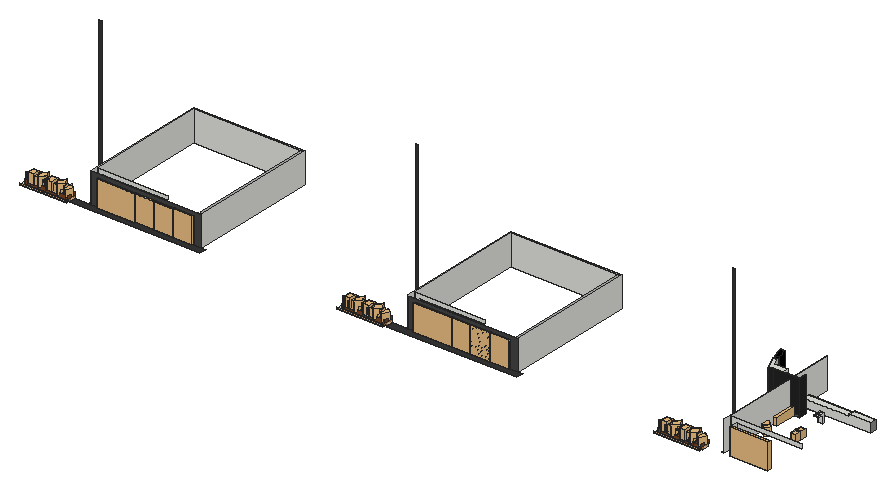
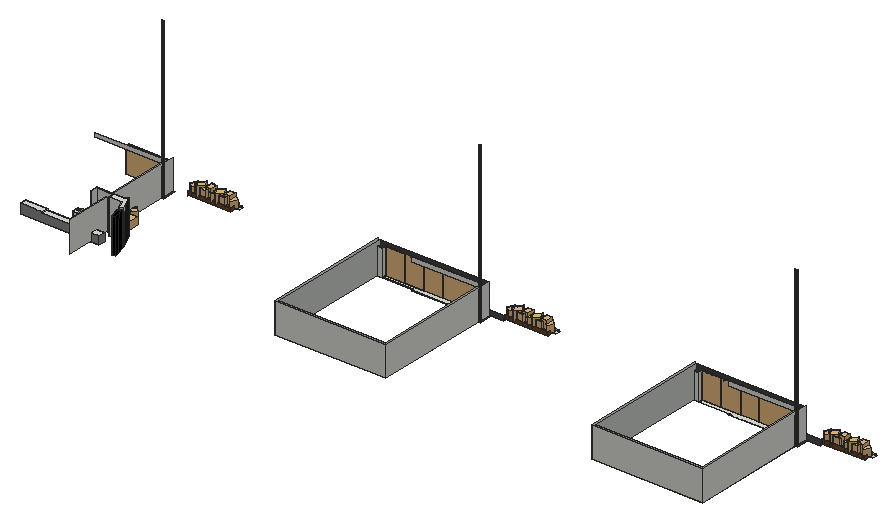
# SketchUp Ruby script. Lengths in inches.
U = 1.inch
M = Sketchup.active_model
def pt(a) = Geom::Point3d.new(a.map { |v| v * U })
def face(e, loops, mat)
  f = e.add_face(loops[0].map { |a| pt(a) })
  loops[1..].each { |l| e.add_face(l.map { |a| pt(a) }).erase! }
  f.material = f.back_material = mat if mat
  f
end
# faces: each face lists its corners as indices into pts; further lists are holes
def faces(e, pts, list, mat = nil) = list.each { |f| face(e, (f[0].is_a?(Array) ? f : [f]).map { |l| l.map { |i| pts[i] } }, mat) }
# xy, xz, yz: faces in a plane at the given z, y or x. An outline is a flat list of corners, or four numbers for a rectangle; further outlines are holes
def ring(l) = l.size == 4 ? [[l[0], l[1]], [l[2], l[1]], [l[2], l[3]], [l[0], l[3]]] : l.each_slice(2).to_a
def flat(e, list, mat, &to3) = list.each { |f| face(e, (f[0].is_a?(Array) ? f : [f]).map { |l| ring(l).map { |u, v| to3.(u, v) } }, mat) }
def xy(e, z, list, mat = nil) = flat(e, list, mat) { |x, y| [x, y, z] }
def xz(e, y, list, mat = nil) = flat(e, list, mat) { |x, z| [x, y, z] }
def yz(e, x, list, mat = nil) = flat(e, list, mat) { |y, z| [x, y, z] }
def lines(e, pts, list) = list.each { |a, b| e.add_line(pt(pts[a]), pt(pts[b])) }
# prism: a flat outline (further loops are holes) pulled along v
def prism(e, loops, v, mat = nil)
  f = face(e, loops, mat); d = Geom::Vector3d.new(v.map { |x| x * U })
  f.pushpull(f.normal.samedirection?(d) ? d.length : -d.length)
end
def box(e, o, s, mat = nil) = prism(e, [[o, [o[0] + s[0], o[1], o[2]], [o[0] + s[0], o[1] + s[1], o[2]], [o[0], o[1] + s[1], o[2]]]], [0, 0, s[2]], mat)
def at(x, y, z, deg = 0) = Geom::Transformation.translation(pt([x, y, z])) * Geom::Transformation.rotation(ORIGIN, Z_AXIS, deg.degrees)
def axes(o, x, y, z) = Geom::Transformation.new([*x, 0, *y, 0, *z, 0, *pt(o).to_a, 1])
def part(name) = M.definitions.add(name)
# library, detail: a bought-in or finely detailed component or shape, given as its bounding box
def library(name, o, s) = part(name).tap { |d| box(d.entities, o, s) }
def detail(e, o, s) = box(e.add_group.entities, o, s)
def put(e, d, t, mat = nil) = e.add_instance(d, t).tap { |i| i.material = mat if mat }
def group(e, t, mat = nil) = e.add_group.tap { |g| g.transformation = t; g.material = mat if mat }.entities
root = M.entities
M.materials.add("Material__1").color = [95, 70, 46]
M.materials.add("Sophie_Shoes2").color = [35, 35, 35]
M.materials.add("Sophie_Skirt").color = [0, 0, 0]
M.materials.add("Stain").color = [141, 140, 139]
M.materials.add("Untitsled-1").color = [96, 91, 93]
M.materials.add("[Basic Tile]").color = [203, 206, 202]
M.materials.add("[Granite Dark Gray]").color = [69, 68, 68]
M.materials.add("[Slate Light Tile]").color = [54, 54, 54]
M.materials.add("[Wood Floor]").color = [224, 152, 88]
M.materials["[Wood Floor]"].alpha = 0.68
M.materials.add("[Wood Veneer 01]").color = [120, 70, 37]
c1 = library("Areca palm plant",[0,0,0],[49.1,36.6,54.46])
c2 = library("Group\#440",[-84.69,-90.07,-0.36],[176.51,175.13,171.4])
c3 = library("Group\#441",[-7.34,-1.2,0],[38.67,35.81,49.04])
c4 = library("Group38\#2",[14.01,28.44,-23.43],[18.58,18.32,38.89])
c5 = library("Group20\#1",[-20.81,-17.08,3.79],[39.86,39.43,37.51])
c6 = part("Group\#443")
put(c6.entities,c1,axes([76.39,-6.2,6.08],[0.56191,0.45017,0],[-0.52986,0.66137,0],[0,0,0.72]))
put(c6.entities,c1,axes([178.2,-6.2,6.08],[0.56191,0.45017,0],[-0.52986,0.66137,0],[0,0,0.72]))
put(c6.entities,c2,axes([163.5,14.93,6.05],[0.08593,-0.04961,0],[0.04961,0.08593,0],[0,0,0.10522]))
put(c6.entities,c3,axes([144.89,24.9375,8],[-0.79,0,0],[0,-0.79,0],[0,0,0.79]))
put(c6.entities,c2,axes([113.57,17.19,6.07],[0.14087,-0.08133,0],[0.08133,0.14087,0],[0,0,0.1725]))
put(c6.entities,c4,axes([235.95,-4.1,28.17],[0,0.8848,0],[-0.94674,0,0],[0,0,0.85826]))
put(c6.entities,c2,axes([190.75,14.93,6.05],[0.08593,-0.04961,0],[0.04961,0.08593,0],[0,0,0.10522]))
put(c6.entities,c2,axes([61.68,14.93,6.05],[0.08593,-0.04961,0],[0.04961,0.08593,0],[0,0,0.10522]))
put(c6.entities,c2,axes([88.93,14.93,6.05],[0.08593,-0.04961,0],[0.04961,0.08593,0],[0,0,0.10522]))
put(c6.entities,c5,axes([154.82,18.97,4.77],[-0.85,0,0],[0,-0.85,0],[0,0,0.85]))
put(c6.entities,c2,axes([41.62,14.93,6.05],[0.08593,-0.04961,0],[0.04961,0.08593,0],[0,0,0.10522]))
put(c6.entities,c2,axes([143.43,14.93,6.05],[0.08593,-0.04961,0],[0.04961,0.08593,0],[0,0,0.10522]))
put(c6.entities,c4,axes([134.14,-4.1,28.17],[0,0.8848,0],[-0.94674,0,0],[0,0,0.85826]))
g1 = group(c6.entities,at(234.8,0,0,90),"[Wood Veneer 01]")
xy(g1,0,[[0,0,6,234.8],[30,0,36,234.8]])
xy(g1,3,[[6,0,30,234.8]])
xy(g1,7,[[6,5,30,229.8]],"Material__1")
xy(g1,15,[[[0,0,36,234.8],[6,5,30,229.8]]])
xz(g1,0,[[0,0,6,0,6,3,30,3,30,0,36,0,36,15,0,15]])
xz(g1,5,[[6,7,30,15]])
xz(g1,229.8,[[6,7,30,15]])
xz(g1,234.8,[[0,0,0,15,36,15,36,0,30,0,30,3,6,3,6,0]])
yz(g1,0,[[0,0,234.8,15]])
yz(g1,6,[[0,0,234.8,3],[5,7,229.8,15]])
yz(g1,30,[[0,0,234.8,3],[5,7,229.8,15]])
yz(g1,36,[[0,0,234.8,15]])
put(c6.entities,c3,axes([43.08,24.9375,8],[-0.79,0,0],[0,-0.79,0],[0,0,0.79]))
put(c6.entities,c2,axes([11.76,17.19,6.07],[0.14087,-0.08133,0],[0.08133,0.14087,0],[0,0,0.1725]))
put(c6.entities,c5,axes([53.01,18.97,4.77],[-0.85,0,0],[0,-0.85,0],[0,0,0.85]))
put(c6.entities,c2,axes([219.01,17.19,6.07],[0.14087,-0.08133,0],[0.08133,0.14087,0],[0,0,0.1725]))
c7 = library("Scandinavian Door w/ Glass Wall\#2",[-41.94,78.85,0],[6.47,62.99,82.68])
c8 = library("Group\#86",[-0.03,0.1,-0.2],[72.93,84.1,29.53])
c9 = library("ch24 wishbone chair by Carl Hansen & Son",[0,0,0],[21.1,19.68,29.02])
c10 = library("Square table",[5.01,5.91,-0.2],[27.56,27.56,29.53])
xy(root,148.4375,[[551.76,589.17,551.76,1096.5,990.19,1096.5,990.19,589.17,956.36,589.17,956.36,608.75,979.42,608.75,979.42,1090.24,558.02,1090.24,558.02,616,578.37,616,578.37,589.17],[578.37,589.17,578.37,616,835.39,616,835.39,608.75,956.36,608.75,956.36,589.17],[1802.38,589.17,1802.38,1096.5,2240.81,1096.5,2240.81,589.17,2206.98,589.17,2206.98,608.75,2230.05,608.75,2230.05,1090.24,1808.65,1090.24,1808.65,616,1829,616,1829,589.17],[1829,589.17,1829,616,2086.01,616,2086.01,608.75,2206.98,608.75,2206.98,589.17]])
xy(root,148.4375,[[492.21,559.875,1005.5,589.17],[1742.84,559.875,2256.12,589.17],[543.03,589.17,551.76,640.11],[1793.65,589.17,1802.38,640.11],[3044.28,589.17,3053.01,640.11]],"[Slate Light Tile]")
xy(root,149.625,[[578.37,589.17,956.36,589.17,956.36,608.75,835.39,608.75,835.39,616,578.37,616],[1829,589.17,2206.98,589.17,2206.98,608.75,2086.01,608.75,2086.01,616,1829,616]])
xy(root,155.3125,[[310,542.125,492.21,559.875],[1560.62,542.125,1742.84,559.875],[2811.25,542.125,2993.46,559.875]])
xz(root,542.125,[[310,155.3125,492.21,161.375],[1560.62,155.3125,1742.84,161.375],[2811.25,155.3125,2993.46,161.375]],"[Wood Floor]")
xz(root,589.17,[[578.37,148.4375,835.39,149.625],[835.39,148.4375,956.36,149.625],[1829,148.4375,2086.01,149.625],[2086.01,148.4375,2206.98,149.625]])
xz(root,589.17,[[551.76,148.4375,578.37,148.4375,578.37,251.46,956.36,251.46,956.36,148.4375,990.19,148.4375,990.19,265.8125,551.76,265.8125],[1802.38,148.4375,1829,148.4375,1829,251.46,2206.98,251.46,2206.98,148.4375,2240.81,148.4375,2240.81,265.8125,1802.38,265.8125]],"[Granite Dark Gray]")
xz(root,608.75,[[835.39,148.4375,956.36,149.625],[956.36,148.4375,979.42,251.46],[2086.01,148.4375,2206.98,149.625],[2206.98,148.4375,2230.05,251.46]])
xz(root,616,[[558.02,148.4375,558.02,268.4375,835.39,268.4375,835.39,251.46,578.37,251.46,578.37,148.4375],[578.37,148.4375,835.39,149.625],[1808.65,148.4375,1808.65,268.4375,2086.01,268.4375,2086.01,251.46,1829,251.46,1829,148.4375],[1829,148.4375,2086.01,149.625],[3059.27,148.4375,3059.27,268.4375,3336.64,268.4375,3336.64,251.46,3079.62,251.46,3079.62,148.4375]])
xz(root,640.11,[[543.03,148.4375,551.76,148.4375,551.76,289.5625,548.32,289.5625,548.32,293,551.76,293,551.76,410.625,549.82,410.625,549.82,413.5,551.76,413.5,551.76,538.1875,550.01,538.1875,550.01,541.1875,551.76,541.1875,551.76,662.4375,549.88,662.4375,549.88,665.9375,551.76,665.9375,551.76,776.0625,543.03,776.0625],[1793.65,148.4375,1802.38,148.4375,1802.38,289.5625,1798.95,289.5625,1798.95,293,1802.38,293,1802.38,410.625,1800.45,410.625,1800.45,413.5,1802.38,413.5,1802.38,538.1875,1800.63,538.1875,1800.63,541.1875,1802.38,541.1875,1802.38,662.4375,1800.51,662.4375,1800.51,665.9375,1802.38,665.9375,1802.38,776.0625,1793.65,776.0625],[3044.28,148.4375,3053.01,148.4375,3053.01,289.5625,3049.57,289.5625,3049.57,293,3053.01,293,3053.01,410.625,3051.07,410.625,3051.07,413.5,3053.01,413.5,3053.01,538.1875,3051.26,538.1875,3051.26,541.1875,3053.01,541.1875,3053.01,662.4375,3051.13,662.4375,3051.13,665.9375,3053.01,665.9375,3053.01,776.0625,3044.28,776.0625]],"[Slate Light Tile]")
xz(root,1090.24,[[558.02,148.4375,979.42,268.4375],[1808.65,148.4375,2230.05,268.4375]])
xz(root,1096.5,[[551.76,148.4375,990.19,268.4375],[1802.38,148.4375,2240.81,268.4375]])
yz(root,492.21,[[559.875,148.4375,589.17,148.4375,589.17,161.375,542.125,161.375,542.125,155.3125,559.875,155.3125]],"[Wood Floor]")
yz(root,551.76,[[589.17,148.4375,640.11,268.4375],[640.11,148.4375,1096.5,268.4375]])
yz(root,558.02,[[616,148.4375,1090.24,268.4375]])
yz(root,578.37,[[589.17,148.4375,616,149.625],[589.17,149.625,616,251.46]])
yz(root,835.39,[[608.75,148.4375,616,149.625]])
yz(root,956.36,[[589.17,148.4375,608.75,149.625],[589.17,149.625,608.75,251.46]])
yz(root,979.42,[[608.75,148.4375,608.75,251.46,595.44,251.46,595.44,268.4375,1090.24,268.4375,1090.24,148.4375]],"[Basic Tile]")
yz(root,990.19,[[589.17,148.4375,1096.5,268.4375]])
yz(root,1742.84,[[559.875,148.4375,589.17,148.4375,589.17,161.375,542.125,161.375,542.125,155.3125,559.875,155.3125]],"[Wood Floor]")
yz(root,1802.38,[[589.17,148.4375,640.11,268.4375],[640.11,148.4375,1096.5,268.4375]])
yz(root,1808.65,[[616,148.4375,1090.24,268.4375]])
yz(root,1829,[[589.17,148.4375,616,149.625],[589.17,149.625,616,251.46]])
yz(root,2086.01,[[608.75,148.4375,616,149.625]])
yz(root,2206.98,[[589.17,148.4375,608.75,149.625],[589.17,149.625,608.75,251.46]])
yz(root,2230.05,[[608.75,148.4375,608.75,251.46,595.44,251.46,595.44,268.4375,1090.24,268.4375,1090.24,148.4375]],"[Basic Tile]")
yz(root,2240.81,[[589.17,148.4375,1096.5,268.4375]])
yz(root,2993.46,[[559.875,148.4375,589.17,148.4375,589.17,161.375,542.125,161.375,542.125,155.3125,559.875,155.3125]],"[Wood Floor]")
yz(root,3053.01,[[589.17,148.4375,640.11,268.4375],[640.11,148.4375,1096.5,268.4375]])
yz(root,3059.27,[[616,148.4375,1090.24,268.4375]])
yz(root,3079.62,[[589.17,148.4375,616,149.625],[589.17,149.625,616,251.46]])
p = [[2949.76,1016.67,148.89],[2952.73,1006.41,148.89]]
lines(root,p,[[0,1]])
put(root,c6,axes([319.12,553.5,156.81],[0.72468,0,0],[0,1,0],[0,0,1]))
put(root,c7,axes([578.37,518.89,378.93],[0,-1.83,0],[0,0,-1.61667],[1.83,0,0]))
put(root,c7,axes([729.67,518.17,380.12],[0,-1.83,0],[0,0,-1.61667],[1.83,0,0]))
put(root,c7,axes([803.93,518.17,380.12],[0,-1.83,0],[0,0,-1.61667],[1.83,0,0]))
put(root,c6,axes([1569.74,553.5,156.81],[0.72468,0,0],[0,1,0],[0,0,1]))
put(root,c7,axes([1829,518.89,378.93],[0,-1.83,0],[0,0,-1.61667],[1.83,0,0]))
put(root,c7,axes([1980.3,518.17,380.12],[0,-1.83,0],[0,0,-1.61667],[1.83,0,0]))
put(root,c7,axes([2054.56,518.17,380.12],[0,-1.83,0],[0,0,-1.61667],[1.83,0,0]))
put(root,c6,axes([2820.37,553.5,156.81],[0.72468,0,0],[0,1,0],[0,0,1]))
g2 = group(root,at(2933.37,971.39,148.89),"Sophie_Skirt")
prism(g2,[[[16.39,45.28,0],[27.93,5.32,0],[13.08,0,0],[5.78,22.42,0],[0,45.28,0]]],[0,0,137.8])
g3 = group(root,at(2951.76,898.55,148.89))
xy(g3,0,[[26.99,0,5.49,42.96,0,58.01,14.86,63.33,26.8,35.09,78.61,35.09,78.61,13.375,141.6,13.375,141.6,37,147.51,37,147.51,7.04,40.37,7.04,40.37,7.47]])
xy(g3,7.875,[[40.37,7.04,147.51,7.47]],"Untitsled-1")
xy(g3,137.8,[[26.99,0,40.37,7.47,147.51,7.47,147.51,37,141.6,37,141.6,13.375,78.61,13.375,78.61,35.09,26.8,35.09,14.86,63.33,0,58.01,5.49,42.96]])
xz(g3,7.04,[[40.37,0,147.51,7.875]],"Untitsled-1")
xz(g3,7.47,[[40.37,7.875,147.51,137.8]],"Sophie_Shoes2")
xz(g3,13.375,[[78.61,0,141.6,137.8]])
xz(g3,35.09,[[26.8,0,78.61,137.8]])
xz(g3,37,[[141.6,0,147.51,137.8]])
yz(g3,40.37,[[7.04,0,7.47,7.875]])
yz(g3,78.61,[[13.375,0,35.09,137.8]])
yz(g3,141.6,[[13.375,0,37,137.8]])
yz(g3,147.51,[[7.04,0,37,0,37,137.8,7.47,137.8,7.47,7.875,7.04,7.875]],"Sophie_Shoes2")
p = [[5.49,42.96,0],[26.99,0,0],[26.99,0,3.9375],[26.99,0,137.8],[5.49,42.96,137.8],[40.37,7.47,0],
  [40.37,7.47,3.9375],[26.8,35.09,0],[14.86,63.33,0],[14.86,63.33,137.8],[26.8,35.09,137.8],[0,58.01,0],
  [0,58.01,137.8],[40.37,7.47,7.875],[40.37,7.47,137.8]]
faces(g3,p,[[0,1,2,3,4],[3,2,6,13,14]],"Sophie_Shoes2")
faces(g3,p,[[5,6,2,1],[7,8,9,10],[11,0,4,12],[8,11,12,9]])
put(root,c8,at(3002.71,821.77,148.89))
put(root,c9,at(3042.9,781.08,148.89,50.338))
put(root,c10,at(3058.875,805.35,148.89,-129.662))
put(root,c9,axes([3068.8,759.73,148.89],[0.63382,0.77348,0],[0.77348,-0.63382,0],[0,0,1]))
put(root,c7,axes([3079.62,518.89,378.93],[0,-1.83,0],[0,0,-1.61667],[1.83,0,0]))
g4 = group(root,at(3159.3,900.11,180.38))
xy(g4,-31.5,[[0,19.69,18.11,26.38]])
xy(g4,0,[[[0,0,18.11,19.69],[1.09,8.35,17.09,13.35]]])
xy(g4,3.9375,[[[0,0,18.11,26.38],[1.09,8.35,17.09,13.35]]])
xz(g4,0,[[0,0,18.11,3.9375]])
xz(g4,8.35,[[1.09,0,17.09,3.9375]])
xz(g4,13.35,[[1.09,0,17.09,3.9375]])
xz(g4,19.69,[[0,-31.5,18.11,0]])
xz(g4,26.38,[[0,-31.5,18.11,3.9375]])
yz(g4,0,[[19.69,-31.5,19.69,0,0,0,0,3.9375,26.38,3.9375,26.38,-31.5]])
yz(g4,1.09,[[8.35,0,13.35,3.9375]])
yz(g4,17.09,[[8.35,0,13.35,3.9375]])
yz(g4,18.11,[[19.69,-31.5,26.38,-31.5,26.38,3.9375,0,3.9375,0,0,19.69,0]])
g5 = group(root,at(2828.42,628.29,148.89))
xy(g5,0,[[190.59,338.75,502.63,364.34]],"Stain")
xy(g5,31.5,[[190.59,338.75,416.02,364.34]])
xy(g5,37.4,[[416.02,338.75,502.63,364.34]])
xz(g5,338.75,[[190.59,0,502.63,0,502.63,37.4,416.02,37.4,416.02,31.5,190.59,31.5]])
xz(g5,364.34,[[190.59,0,190.59,31.5,416.02,31.5,416.02,37.4,502.63,37.4,502.63,0]],"Stain")
yz(g5,190.59,[[338.75,0,364.34,31.5]],"Stain")
yz(g5,416.02,[[338.75,31.5,364.34,37.4]])
yz(g5,502.63,[[338.75,0,364.34,37.4]],"Stain")
put(root,c9,axes([3186.58,796.07,148.89],[0.00287,-1,0],[-1,-0.00287,0],[0,0,1]))
put(root,c9,axes([3186.58,823.08,148.89],[0.00287,-1,0],[-1,-0.00287,0],[0,0,1]))
